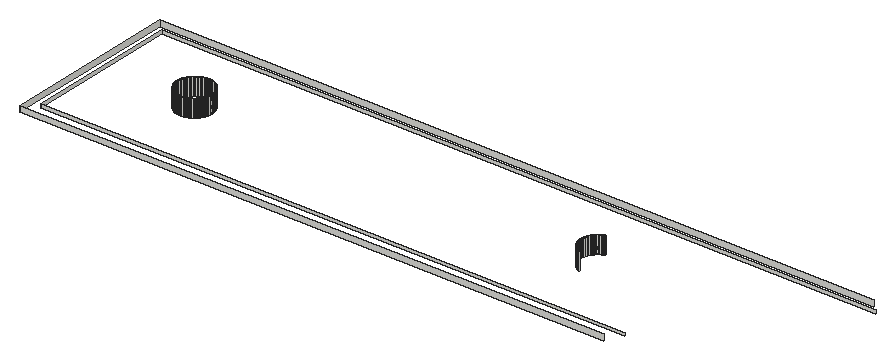
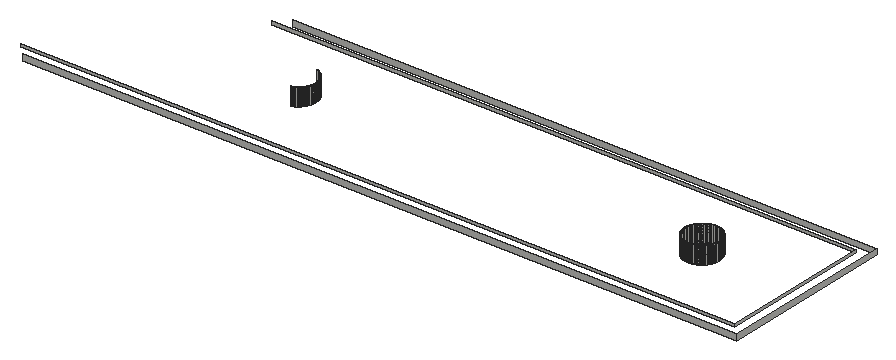
# SketchUp Ruby script. Lengths in inches.
U = 1.inch
M = Sketchup.active_model
def pt(a) = Geom::Point3d.new(a.map { |v| v * U })
def face(e, loops, mat)
  f = e.add_face(loops[0].map { |a| pt(a) })
  loops[1..].each { |l| e.add_face(l.map { |a| pt(a) }).erase! }
  f.material = f.back_material = mat if mat
  f
end
# faces: each face lists its corners as indices into pts; further lists are holes
def faces(e, pts, list, mat = nil) = list.each { |f| face(e, (f[0].is_a?(Array) ? f : [f]).map { |l| l.map { |i| pts[i] } }, mat) }
# xy, xz, yz: faces in a plane at the given z, y or x. An outline is a flat list of corners, or four numbers for a rectangle; further outlines are holes
def ring(l) = l.size == 4 ? [[l[0], l[1]], [l[2], l[1]], [l[2], l[3]], [l[0], l[3]]] : l.each_slice(2).to_a
def flat(e, list, mat, &to3) = list.each { |f| face(e, (f[0].is_a?(Array) ? f : [f]).map { |l| ring(l).map { |u, v| to3.(u, v) } }, mat) }
def xy(e, z, list, mat = nil) = flat(e, list, mat) { |x, y| [x, y, z] }
def xz(e, y, list, mat = nil) = flat(e, list, mat) { |x, z| [x, y, z] }
def yz(e, x, list, mat = nil) = flat(e, list, mat) { |y, z| [x, y, z] }
def lines(e, pts, list) = list.each { |a, b| e.add_line(pt(pts[a]), pt(pts[b])) }
# prism: a flat outline (further loops are holes) pulled along v
def prism(e, loops, v, mat = nil)
  f = face(e, loops, mat); d = Geom::Vector3d.new(v.map { |x| x * U })
  f.pushpull(f.normal.samedirection?(d) ? d.length : -d.length)
end
def box(e, o, s, mat = nil) = prism(e, [[o, [o[0] + s[0], o[1], o[2]], [o[0] + s[0], o[1] + s[1], o[2]], [o[0], o[1] + s[1], o[2]]]], [0, 0, s[2]], mat)
def at(x, y, z, deg = 0) = Geom::Transformation.translation(pt([x, y, z])) * Geom::Transformation.rotation(ORIGIN, Z_AXIS, deg.degrees)
def axes(o, x, y, z) = Geom::Transformation.new([*x, 0, *y, 0, *z, 0, *pt(o).to_a, 1])
def part(name) = M.definitions.add(name)
# library, detail: a bought-in or finely detailed component or shape, given as its bounding box
def library(name, o, s) = part(name).tap { |d| box(d.entities, o, s) }
def detail(e, o, s) = box(e.add_group.entities, o, s)
def put(e, d, t, mat = nil) = e.add_instance(d, t).tap { |i| i.material = mat if mat }
def group(e, t, mat = nil) = e.add_group.tap { |g| g.transformation = t; g.material = mat if mat }.entities
root = M.entities
xz(root,173,[[33,107.5,133.5,108.5]])
xz(root,175,[[35,108,135.5,108.5]])
xz(root,185,[[50.84,108,50.92,111],[50.92,108,51,111],[51,108,51.08,111],[51.08,108,51.16,111]])
xz(root,191,[[50.84,108,50.92,111],[50.92,108,51,111],[51,108,51.08,111],[51.08,108,51.16,111]])
xz(root,201,[[35,108,158,108.5]])
xz(root,203,[[33,107.5,156,108.5]])
yz(root,33,[[173,107.5,203,108.5]])
yz(root,35,[[175,108,201,108.5]])
yz(root,48,[[187.84,108,187.92,111],[187.92,108,188,111],[188,108,188.08,111],[188.08,108,188.16,111]])
yz(root,54,[[187.84,108,187.92,111],[187.92,108,188,111],[188,108,188.08,111],[188.08,108,188.16,111]])
yz(root,117.5,[[187.84,108,187.92,111],[187.92,108,188,111],[188,108,188.08,111],[188.08,108,188.16,111]])
p = [[50.53,185.04,108],[50.45,185.05,108],[50.45,185.05,111],[50.53,185.04,111],[50.61,185.03,108],[50.61,185.03,111],
  [50.6875,185.02,108],[50.6875,185.02,111],[50.76,185.01,108],[50.76,185.01,111],[50.84,185,108],[50.84,185,111],
  [51.24,185.01,108],[51.16,185,108],[51.16,185,111],[51.24,185.01,111],[51.3125,185.02,108],[51.3125,185.02,111],
  [51.39,185.03,108],[51.39,185.03,111],[51.47,185.04,108],[51.47,185.04,111],[51.55,185.05,108],[51.55,185.05,111],
  [50.07,185.15,108],[50,185.17,108],[50,185.17,111],[50.07,185.15,111],[50.15,185.125,108],[50.15,185.125,111],
  [50.22,185.1,108],[50.22,185.1,111],[50.3,185.08,108],[50.3,185.08,111],[50.375,185.07,108],[50.375,185.07,111],
  [51.625,185.07,108],[51.625,185.07,111],[51.7,185.08,108],[51.7,185.08,111],[51.78,185.1,108],[51.78,185.1,111],
  [51.85,185.125,108],[51.85,185.125,111],[51.93,185.15,108],[51.93,185.15,111],[52,185.17,108],[52,185.17,111],
  [119.57,185.15,108],[119.5,185.17,108],[119.5,185.17,111],[119.57,185.15,111],[49.85,185.23,108],[49.78,185.26,108],
  [49.78,185.26,111],[49.85,185.23,111],[49.92,185.2,108],[49.92,185.2,111],[52.08,185.2,108],[52.08,185.2,111],
  [52.15,185.23,108],[52.15,185.23,111],[52.22,185.26,108],[52.22,185.26,111],[119.35,185.23,108],[119.28,185.26,108],
  [119.28,185.26,111],[119.35,185.23,111],[119.42,185.2,108],[119.42,185.2,111],[49.64,185.33,108],[49.57,185.36,108],
  [49.57,185.36,111],[49.64,185.33,111],[49.71,185.29,108],[49.71,185.29,111],[52.29,185.29,108],[52.29,185.29,111],
  [52.36,185.33,108],[52.36,185.33,111],[52.43,185.36,108],[52.43,185.36,111],[119.14,185.33,108],[119.07,185.36,108],
  [119.07,185.36,111],[119.14,185.33,111],[119.21,185.29,108],[119.21,185.29,111],[49.43,185.44,108],[49.37,185.48,108],
  [49.37,185.48,111],[49.43,185.44,111],[49.5,185.4,108],[49.5,185.4,111],[52.5,185.4,108],[52.5,185.4,111],
  [52.57,185.44,108],[52.57,185.44,111],[52.63,185.48,108],[52.63,185.48,111],[118.93,185.44,108],[118.87,185.48,108],
  [118.87,185.48,111],[118.93,185.44,111],[119,185.4,108],[119,185.4,111],[49.3,185.53,108],[49.24,185.57,108],
  [49.24,185.57,111],[49.3,185.53,111],[52.7,185.53,108],[52.7,185.53,111],[52.76,185.57,108],[52.76,185.57,111],
  [118.8,185.53,108],[118.74,185.57,108],[118.74,185.57,111],[118.8,185.53,111],[49.17,185.62,108],[49.11,185.67,108],
  [49.11,185.67,111],[49.17,185.62,111],[52.83,185.62,108],[52.83,185.62,111],[52.89,185.67,108],[52.89,185.67,111],
  [118.67,185.62,108],[118.61,185.67,108],[118.61,185.67,111],[118.67,185.62,111],[49.05,185.72,108],[48.99,185.77,108],
  [48.99,185.77,111],[49.05,185.72,111],[52.95,185.72,108],[52.95,185.72,111],[53.01,185.77,108],[53.01,185.77,111],
  [118.55,185.72,108],[118.49,185.77,108],[118.49,185.77,111],[118.55,185.72,111],[48.93,185.82,108],[48.88,185.88,108],
  [48.88,185.88,111],[48.93,185.82,111],[53.07,185.82,108],[53.07,185.82,111],[53.12,185.88,108],[53.12,185.88,111],
  [118.43,185.82,108],[118.38,185.88,108],[118.38,185.88,111],[118.43,185.82,111],[48.82,185.93,108],[48.77,185.99,108],
  [48.77,185.99,111],[48.82,185.93,111],[53.18,185.93,108],[53.18,185.93,111],[53.23,185.99,108],[53.23,185.99,111],
  [118.32,185.93,108],[118.27,185.99,108],[118.27,185.99,111],[118.32,185.93,111],[48.72,186.05,108],[48.72,186.05,111],
  [53.28,186.05,108],[53.28,186.05,111],[118.22,186.05,108],[118.22,186.05,111],[48.67,186.11,108],[48.62,186.17,108],
  [48.62,186.17,111],[48.67,186.11,111],[53.33,186.11,108],[53.33,186.11,111],[53.38,186.17,108],[53.38,186.17,111],
  [118.17,186.11,108],[118.12,186.17,108],[118.12,186.17,111],[118.17,186.11,111],[48.57,186.24,108],[48.53,186.3,108],
  [48.53,186.3,111],[48.57,186.24,111],[53.43,186.24,108],[53.43,186.24,111],[53.47,186.3,108],[53.47,186.3,111],
  [118.07,186.24,108],[118.03,186.3,108],[118.03,186.3,111],[118.07,186.24,111],[48.48,186.37,108],[48.48,186.37,111],
  [53.52,186.37,108],[53.52,186.37,111],[117.98,186.37,108],[117.98,186.37,111],[48.44,186.43,108],[48.4,186.5,108],
  [48.4,186.5,111],[48.44,186.43,111],[53.56,186.43,108],[53.56,186.43,111],[53.6,186.5,108],[53.6,186.5,111],
  [117.94,186.43,108],[117.9,186.5,108],[117.9,186.5,111],[117.94,186.43,111],[48.36,186.57,108],[48.36,186.57,111],
  [53.64,186.57,108],[53.64,186.57,111],[117.86,186.57,108],[117.86,186.57,111],[48.33,186.64,108],[48.29,186.71,108],
  [48.29,186.71,111],[48.33,186.64,111],[53.67,186.64,108],[53.67,186.64,111],[53.71,186.71,108],[53.71,186.71,111],
  [117.83,186.64,108],[117.79,186.71,108],[117.79,186.71,111],[117.83,186.64,111],[48.26,186.78,108],[48.26,186.78,111],
  [53.74,186.78,108],[53.74,186.78,111],[117.76,186.78,108],[117.76,186.78,111],[48.23,186.85,108],[48.23,186.85,111],
  [53.77,186.85,108],[53.77,186.85,111],[117.73,186.85,108],[117.73,186.85,111],[48.2,186.92,108],[48.17,187,108],
  [48.17,187,111],[48.2,186.92,111],[53.8,186.92,108],[53.8,186.92,111],[53.83,187,108],[53.83,187,111],
  [117.7,186.92,108],[117.67,187,108],[117.67,187,111],[117.7,186.92,111],[48.15,187.07,108],[48.15,187.07,111],
  [53.85,187.07,108],[53.85,187.07,111],[117.65,187.07,108],[117.65,187.07,111],[48.125,187.15,108],[48.1,187.22,108],
  [48.1,187.22,111],[48.125,187.15,111],[53.875,187.15,108],[53.875,187.15,111],[53.9,187.22,108],[53.9,187.22,111],
  [117.625,187.15,108],[117.6,187.22,108],[117.6,187.22,111],[117.625,187.15,111],[48.08,187.3,108],[48.08,187.3,111],
  [53.92,187.3,108],[53.92,187.3,111],[117.58,187.3,108],[117.58,187.3,111],[48.07,187.375,108],[48.07,187.375,111],
  [53.93,187.375,108],[53.93,187.375,111],[117.57,187.375,108],[117.57,187.375,111],[48.05,187.45,108],[48.05,187.45,111],
  [53.95,187.45,108],[53.95,187.45,111],[117.55,187.45,108],[117.55,187.45,111],[48.04,187.53,108],[48.03,187.61,108],
  [48.03,187.61,111],[48.04,187.53,111],[53.96,187.53,108],[53.96,187.53,111],[53.97,187.61,108],[53.97,187.61,111],
  [117.54,187.53,108],[117.53,187.61,108],[117.53,187.61,111],[117.54,187.53,111],[48.02,187.6875,108],[48.02,187.6875,111],
  [53.98,187.6875,108],[53.98,187.6875,111],[117.52,187.6875,108],[117.52,187.6875,111],[48.01,187.76,108],[48.01,187.76,111],
  [53.99,187.76,108],[53.99,187.76,111],[117.51,187.76,108],[117.51,187.76,111],[48,187.84,108],[48,187.84,111],
  [54,187.84,108],[54,187.84,111],[117.5,187.84,108],[117.5,187.84,111],[48,188.16,108],[48.01,188.24,108],
  [48.01,188.24,111],[48,188.16,111],[48.02,188.3125,108],[48.02,188.3125,111],[53.98,188.3125,108],[53.99,188.24,108],
  [53.99,188.24,111],[53.98,188.3125,111],[54,188.16,108],[54,188.16,111],[117.5,188.16,108],[117.51,188.24,108],
  [117.51,188.24,111],[117.5,188.16,111],[117.52,188.3125,108],[117.52,188.3125,111],[48.03,188.39,108],[48.03,188.39,111],
  [53.97,188.39,108],[53.97,188.39,111],[117.53,188.39,108],[117.53,188.39,111],[48.04,188.47,108],[48.04,188.47,111],
  [53.96,188.47,108],[53.96,188.47,111],[117.54,188.47,108],[117.54,188.47,111],[48.05,188.55,108],[48.05,188.55,111],
  [48.07,188.625,108],[48.07,188.625,111],[53.93,188.625,108],[53.95,188.55,108],[53.95,188.55,111],[53.93,188.625,111],
  [117.55,188.55,108],[117.55,188.55,111],[117.57,188.625,108],[117.57,188.625,111],[48.08,188.7,108],[48.08,188.7,111],
  [53.92,188.7,108],[53.92,188.7,111],[117.58,188.7,108],[117.58,188.7,111],[48.1,188.78,108],[48.1,188.78,111],
  [53.9,188.78,108],[53.9,188.78,111],[117.6,188.78,108],[117.6,188.78,111],[48.125,188.85,108],[48.125,188.85,111],
  [53.875,188.85,108],[53.875,188.85,111],[117.625,188.85,108],[117.625,188.85,111],[48.15,188.93,108],[48.15,188.93,111],
  [48.17,189,108],[48.17,189,111],[53.83,189,108],[53.85,188.93,108],[53.85,188.93,111],[53.83,189,111],
  [117.65,188.93,108],[117.65,188.93,111],[117.67,189,108],[117.67,189,111],[48.2,189.08,108],[48.2,189.08,111],
  [53.8,189.08,108],[53.8,189.08,111],[117.7,189.08,108],[117.7,189.08,111],[48.23,189.15,108],[48.23,189.15,111],
  [48.26,189.22,108],[48.26,189.22,111],[53.74,189.22,108],[53.77,189.15,108],[53.77,189.15,111],[53.74,189.22,111],
  [117.73,189.15,108],[117.73,189.15,111],[117.76,189.22,108],[117.76,189.22,111],[48.29,189.29,108],[48.29,189.29,111],
  [53.71,189.29,108],[53.71,189.29,111],[117.79,189.29,108],[117.79,189.29,111],[48.33,189.36,108],[48.33,189.36,111],
  [53.67,189.36,108],[53.67,189.36,111],[117.83,189.36,108],[117.83,189.36,111],[48.36,189.43,108],[48.36,189.43,111],
  [48.4,189.5,108],[48.4,189.5,111],[53.6,189.5,108],[53.64,189.43,108],[53.64,189.43,111],[53.6,189.5,111],
  [117.86,189.43,108],[117.86,189.43,111],[117.9,189.5,108],[117.9,189.5,111],[48.44,189.57,108],[48.44,189.57,111],
  [53.56,189.57,108],[53.56,189.57,111],[117.94,189.57,108],[117.94,189.57,111],[48.48,189.63,108],[48.48,189.63,111],
  [48.53,189.7,108],[48.53,189.7,111],[53.47,189.7,108],[53.52,189.63,108],[53.52,189.63,111],[53.47,189.7,111],
  [117.98,189.63,108],[117.98,189.63,111],[118.03,189.7,108],[118.03,189.7,111],[48.57,189.76,108],[48.57,189.76,111],
  [53.43,189.76,108],[53.43,189.76,111],[118.07,189.76,108],[118.07,189.76,111],[48.62,189.83,108],[48.62,189.83,111],
  [48.67,189.89,108],[48.67,189.89,111],[53.33,189.89,108],[53.38,189.83,108],[53.38,189.83,111],[53.33,189.89,111],
  [118.12,189.83,108],[118.12,189.83,111],[118.17,189.89,108],[118.17,189.89,111],[48.72,189.95,108],[48.72,189.95,111],
  [48.77,190.01,108],[48.77,190.01,111],[53.23,190.01,108],[53.28,189.95,108],[53.28,189.95,111],[53.23,190.01,111],
  [118.22,189.95,108],[118.22,189.95,111],[118.27,190.01,108],[118.27,190.01,111],[48.82,190.07,108],[48.82,190.07,111],
  [53.18,190.07,108],[53.18,190.07,111],[118.32,190.07,108],[118.32,190.07,111],[48.88,190.12,108],[48.88,190.12,111],
  [48.93,190.18,108],[48.93,190.18,111],[53.07,190.18,108],[53.12,190.12,108],[53.12,190.12,111],[53.07,190.18,111],
  [118.38,190.12,108],[118.38,190.12,111],[118.43,190.18,108],[118.43,190.18,111],[48.99,190.23,108],[48.99,190.23,111],
  [49.05,190.28,108],[49.05,190.28,111],[52.95,190.28,108],[53.01,190.23,108],[53.01,190.23,111],[52.95,190.28,111],
  [118.49,190.23,108],[118.49,190.23,111],[118.55,190.28,108],[118.55,190.28,111],[49.11,190.33,108],[49.11,190.33,111],
  [49.17,190.38,108],[49.17,190.38,111],[52.83,190.38,108],[52.89,190.33,108],[52.89,190.33,111],[52.83,190.38,111],
  [118.61,190.33,108],[118.61,190.33,111],[118.67,190.38,108],[118.67,190.38,111],[49.24,190.43,108],[49.24,190.43,111],
  [49.3,190.47,108],[49.3,190.47,111],[52.7,190.47,108],[52.76,190.43,108],[52.76,190.43,111],[52.7,190.47,111],
  [118.74,190.43,108],[118.74,190.43,111],[118.8,190.47,108],[118.8,190.47,111],[49.37,190.52,108],[49.37,190.52,111],
  [49.43,190.56,108],[49.43,190.56,111],[52.57,190.56,108],[52.63,190.52,108],[52.63,190.52,111],[52.57,190.56,111],
  [118.87,190.52,108],[118.87,190.52,111],[118.93,190.56,108],[118.93,190.56,111],[49.5,190.6,108],[49.5,190.6,111],
  [49.57,190.64,108],[49.57,190.64,111],[49.64,190.67,108],[49.64,190.67,111],[52.36,190.67,108],[52.43,190.64,108],
  [52.43,190.64,111],[52.36,190.67,111],[52.5,190.6,108],[52.5,190.6,111],[119,190.6,108],[119,190.6,111],
  [119.07,190.64,108],[119.07,190.64,111],[119.14,190.67,108],[119.14,190.67,111],[49.71,190.71,108],[49.71,190.71,111],
  [49.78,190.74,108],[49.78,190.74,111],[49.85,190.77,108],[49.85,190.77,111],[52.15,190.77,108],[52.22,190.74,108],
  [52.22,190.74,111],[52.15,190.77,111],[52.29,190.71,108],[52.29,190.71,111],[119.21,190.71,108],[119.21,190.71,111],
  [119.28,190.74,108],[119.28,190.74,111],[119.35,190.77,108],[119.35,190.77,111],[49.92,190.8,108],[49.92,190.8,111],
  [50,190.83,108],[50,190.83,111],[50.07,190.85,108],[50.07,190.85,111],[51.93,190.85,108],[52,190.83,108],
  [52,190.83,111],[51.93,190.85,111],[52.08,190.8,108],[52.08,190.8,111],[119.42,190.8,108],[119.42,190.8,111],
  [119.5,190.83,108],[119.5,190.83,111],[119.57,190.85,108],[119.57,190.85,111],[50.15,190.875,108],[50.15,190.875,111],
  [50.22,190.9,108],[50.22,190.9,111],[50.3,190.92,108],[50.3,190.92,111],[50.375,190.93,108],[50.375,190.93,111],
  [50.45,190.95,108],[50.45,190.95,111],[50.53,190.96,108],[50.53,190.96,111],[51.47,190.96,108],[51.55,190.95,108],
  [51.55,190.95,111],[51.47,190.96,111],[51.625,190.93,108],[51.625,190.93,111],[51.7,190.92,108],[51.7,190.92,111],
  [51.78,190.9,108],[51.78,190.9,111],[51.85,190.875,108],[51.85,190.875,111],[50.61,190.97,108],[50.61,190.97,111],
  [50.6875,190.98,108],[50.6875,190.98,111],[50.76,190.99,108],[50.76,190.99,111],[50.84,191,108],[50.84,191,111],
  [51.16,191,108],[51.24,190.99,108],[51.24,190.99,111],[51.16,191,111],[51.3125,190.98,108],[51.3125,190.98,111],
  [51.39,190.97,108],[51.39,190.97,111]]
faces(root,p,[[0,1,2,3],[4,0,3,5],[6,4,5,7],[8,6,7,9],[10,8,9,11],[12,13,14,15],[16,12,15,17],[18,16,17,19],
  [20,18,19,21],[22,20,21,23],[24,25,26,27],[28,24,27,29],[30,28,29,31],[32,30,31,33],[34,32,33,35],[1,34,35,2],
  [36,22,23,37],[38,36,37,39],[40,38,39,41],[42,40,41,43],[44,42,43,45],[46,44,45,47],[48,49,50,51],[52,53,54,55],
  [56,52,55,57],[25,56,57,26],[58,46,47,59],[60,58,59,61],[62,60,61,63],[64,65,66,67],[68,64,67,69],[49,68,69,50],
  [70,71,72,73],[74,70,73,75],[53,74,75,54],[76,62,63,77],[78,76,77,79],[80,78,79,81],[82,83,84,85],[86,82,85,87],
  [65,86,87,66],[88,89,90,91],[92,88,91,93],[71,92,93,72],[94,80,81,95],[96,94,95,97],[98,96,97,99],[100,101,102,103],
  [104,100,103,105],[83,104,105,84],[106,107,108,109],[89,106,109,90],[110,98,99,111],[112,110,111,113],[114,115,116,117],[101,114,117,102],
  [118,119,120,121],[107,118,121,108],[122,112,113,123],[124,122,123,125],[126,127,128,129],[115,126,129,116],[130,131,132,133],[119,130,133,120],
  [134,124,125,135],[136,134,135,137],[138,139,140,141],[127,138,141,128],[142,143,144,145],[131,142,145,132],[146,136,137,147],[148,146,147,149],
  [150,151,152,153],[139,150,153,140],[154,155,156,157],[143,154,157,144],[158,148,149,159],[160,158,159,161],[162,163,164,165],[151,162,165,152],
  [155,166,167,156],[168,160,161,169],[163,170,171,164],[172,173,174,175],[166,172,175,167],[176,168,169,177],[178,176,177,179],[180,181,182,183],
  [170,180,183,171],[184,185,186,187],[173,184,187,174],[188,178,179,189],[190,188,189,191],[192,193,194,195],[181,192,195,182],[185,196,197,186],
  [198,190,191,199],[193,200,201,194],[202,203,204,205],[196,202,205,197],[206,198,199,207],[208,206,207,209],[210,211,212,213],[200,210,213,201],
  [203,214,215,204],[216,208,209,217],[211,218,219,212],[220,221,222,223],[214,220,223,215],[224,216,217,225],[226,224,225,227],[228,229,230,231],
  [218,228,231,219],[221,232,233,222],[234,226,227,235],[229,236,237,230],[232,238,239,233],[240,234,235,241],[236,242,243,237],[244,245,246,247],
  [238,244,247,239],[248,240,241,249],[250,248,249,251],[252,253,254,255],[242,252,255,243],[245,256,257,246],[258,250,251,259],[253,260,261,254],
  [262,263,264,265],[256,262,265,257],[266,258,259,267],[268,266,267,269],[270,271,272,273],[260,270,273,261],[263,274,275,264],[276,268,269,277],
  [271,278,279,272],[274,280,281,275],[282,276,277,283],[278,284,285,279],[280,286,287,281],[288,282,283,289],[284,290,291,285],[292,293,294,295],
  [286,292,295,287],[296,288,289,297],[298,296,297,299],[300,301,302,303],[290,300,303,291],[293,304,305,294],[306,298,299,307],[301,308,309,302],
  [304,310,311,305],[312,306,307,313],[308,314,315,309],[310,316,317,311],[318,312,313,319],[314,320,321,315],[322,323,324,325],[323,326,327,324],
  [328,329,330,331],[329,332,333,330],[334,335,336,337],[335,338,339,336],[326,340,341,327],[342,328,331,343],[338,344,345,339],[340,346,347,341],
  [348,342,343,349],[344,350,351,345],[346,352,353,347],[352,354,355,353],[356,357,358,359],[357,348,349,358],[350,360,361,351],[360,362,363,361],
  [354,364,365,355],[366,356,359,367],[362,368,369,363],[364,370,371,365],[372,366,367,373],[368,374,375,369],[370,376,377,371],[378,372,373,379],
  [374,380,381,375],[376,382,383,377],[382,384,385,383],[386,387,388,389],[387,378,379,388],[380,390,391,381],[390,392,393,391],[384,394,395,385],
  [396,386,389,397],[392,398,399,393],[394,400,401,395],[400,402,403,401],[404,405,406,407],[405,396,397,406],[398,408,409,399],[408,410,411,409],
  [402,412,413,403],[414,404,407,415],[410,416,417,411],[412,418,419,413],[420,414,415,421],[416,422,423,417],[418,424,425,419],[424,426,427,425],
  [428,429,430,431],[429,420,421,430],[422,432,433,423],[432,434,435,433],[426,436,437,427],[438,428,431,439],[434,440,441,435],[436,442,443,437],
  [442,444,445,443],[446,447,448,449],[447,438,439,448],[440,450,451,441],[450,452,453,451],[444,454,455,445],[456,446,449,457],[452,458,459,453],
  [454,460,461,455],[460,462,463,461],[464,465,466,467],[465,456,457,466],[458,468,469,459],[468,470,471,469],[462,472,473,463],[472,474,475,473],
  [476,477,478,479],[477,464,467,478],[470,480,481,471],[480,482,483,481],[474,484,485,475],[486,476,479,487],[482,488,489,483],[484,490,491,485],
  [490,492,493,491],[494,495,496,497],[495,486,487,496],[488,498,499,489],[498,500,501,499],[492,502,503,493],[502,504,505,503],[506,507,508,509],
  [507,494,497,508],[500,510,511,501],[510,512,513,511],[504,514,515,505],[514,516,517,515],[518,519,520,521],[519,506,509,520],[512,522,523,513],
  [522,524,525,523],[516,526,527,517],[526,528,529,527],[530,531,532,533],[531,518,521,532],[524,534,535,525],[534,536,537,535],[528,538,539,529],
  [538,540,541,539],[542,543,544,545],[543,530,533,544],[536,546,547,537],[546,548,549,547],[540,550,551,541],[550,552,553,551],[552,554,555,553],
  [556,557,558,559],[557,560,561,558],[560,542,545,561],[548,562,563,549],[562,564,565,563],[564,566,567,565],[554,568,569,555],[568,570,571,569],
  [570,572,573,571],[574,575,576,577],[575,578,579,576],[578,556,559,579],[566,580,581,567],[580,582,583,581],[582,584,585,583],[572,586,587,573],
  [586,588,589,587],[588,590,591,589],[592,593,594,595],[593,596,597,594],[596,574,577,597],[584,598,599,585],[598,600,601,599],[600,602,603,601],
  [590,604,605,591],[604,606,607,605],[606,608,609,607],[608,610,611,609],[610,612,613,611],[612,614,615,613],[616,617,618,619],[617,620,621,618],
  [620,622,623,621],[622,624,625,623],[624,626,627,625],[626,592,595,627],[614,628,629,615],[628,630,631,629],[630,632,633,631],[632,634,635,633],
  [636,637,638,639],[637,640,641,638],[640,642,643,641],[642,616,619,643]])
